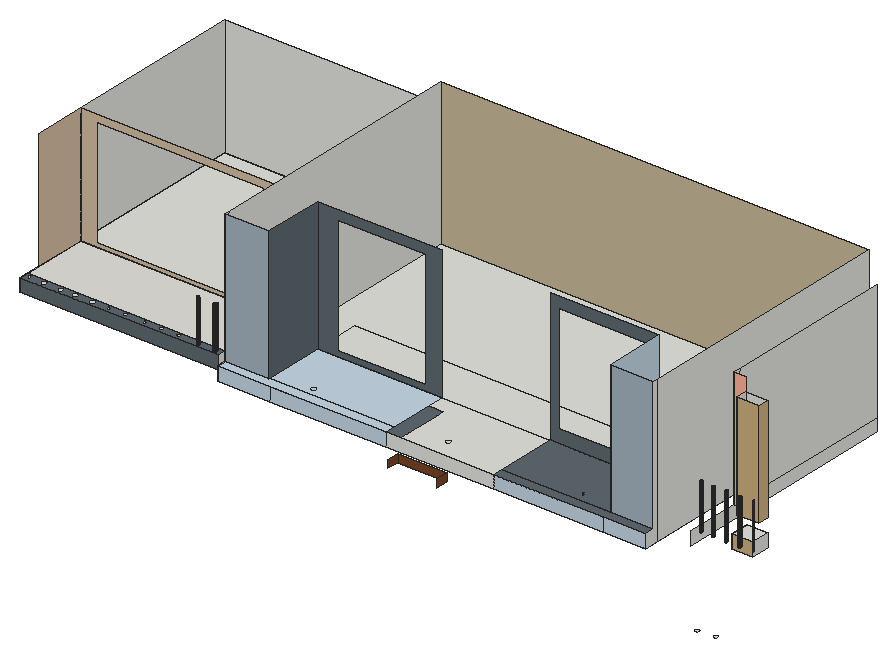
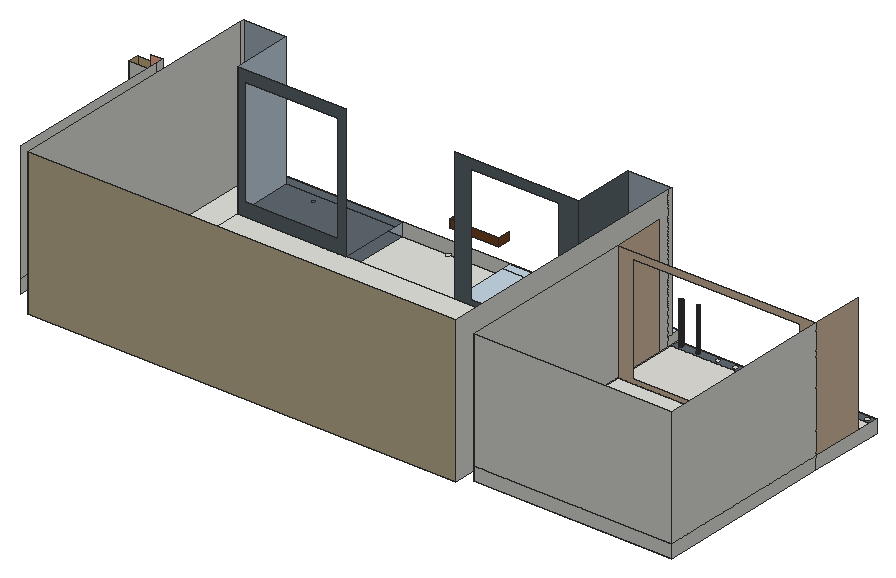
# SketchUp Ruby script. Lengths in inches.
U = 1.inch
M = Sketchup.active_model
def pt(a) = Geom::Point3d.new(a.map { |v| v * U })
def face(e, loops, mat)
  f = e.add_face(loops[0].map { |a| pt(a) })
  loops[1..].each { |l| e.add_face(l.map { |a| pt(a) }).erase! }
  f.material = f.back_material = mat if mat
  f
end
# faces: each face lists its corners as indices into pts; further lists are holes
def faces(e, pts, list, mat = nil) = list.each { |f| face(e, (f[0].is_a?(Array) ? f : [f]).map { |l| l.map { |i| pts[i] } }, mat) }
# xy, xz, yz: faces in a plane at the given z, y or x. An outline is a flat list of corners, or four numbers for a rectangle; further outlines are holes
def ring(l) = l.size == 4 ? [[l[0], l[1]], [l[2], l[1]], [l[2], l[3]], [l[0], l[3]]] : l.each_slice(2).to_a
def flat(e, list, mat, &to3) = list.each { |f| face(e, (f[0].is_a?(Array) ? f : [f]).map { |l| ring(l).map { |u, v| to3.(u, v) } }, mat) }
def xy(e, z, list, mat = nil) = flat(e, list, mat) { |x, y| [x, y, z] }
def xz(e, y, list, mat = nil) = flat(e, list, mat) { |x, z| [x, y, z] }
def yz(e, x, list, mat = nil) = flat(e, list, mat) { |y, z| [x, y, z] }
def lines(e, pts, list) = list.each { |a, b| e.add_line(pt(pts[a]), pt(pts[b])) }
# prism: a flat outline (further loops are holes) pulled along v
def prism(e, loops, v, mat = nil)
  f = face(e, loops, mat); d = Geom::Vector3d.new(v.map { |x| x * U })
  f.pushpull(f.normal.samedirection?(d) ? d.length : -d.length)
end
def box(e, o, s, mat = nil) = prism(e, [[o, [o[0] + s[0], o[1], o[2]], [o[0] + s[0], o[1] + s[1], o[2]], [o[0], o[1] + s[1], o[2]]]], [0, 0, s[2]], mat)
def at(x, y, z, deg = 0) = Geom::Transformation.translation(pt([x, y, z])) * Geom::Transformation.rotation(ORIGIN, Z_AXIS, deg.degrees)
def axes(o, x, y, z) = Geom::Transformation.new([*x, 0, *y, 0, *z, 0, *pt(o).to_a, 1])
def part(name) = M.definitions.add(name)
# library, detail: a bought-in or finely detailed component or shape, given as its bounding box
def library(name, o, s) = part(name).tap { |d| box(d.entities, o, s) }
def detail(e, o, s) = box(e.add_group.entities, o, s)
def put(e, d, t, mat = nil) = e.add_instance(d, t).tap { |i| i.material = mat if mat }
def group(e, t, mat = nil) = e.add_group.tap { |g| g.transformation = t; g.material = mat if mat }.entities
root = M.entities
M.materials.add("[Color B02]").color = [255, 178, 153]
M.materials.add("[Formica Laminate Dark]").color = [50, 53, 60]
M.materials.add("[Formica Laminate Light]").color = [213, 189, 164]
M.materials.add("[Formica Speckled Grey]").color = [94, 105, 111]
M.materials.add("[Marble Carrara Gold Floor Tile]").color = [225, 223, 217]
M.materials.add("[Quartz Light Brown]").color = [199, 184, 152]
M.materials.add("[Terrazzo Light Blue]1").color = [165, 180, 191]
M.materials.add("[Terrazzo Light Blue]2").color = [196, 214, 227]
M.materials.add("[Wood Floor Light]").color = [204, 176, 127]
M.materials.add("[Wood Veneer 01]2").color = [120, 70, 37]
xy(root,184.1875,[[619.39,128.83,619.78,128.89,620.14,129.04,620.45,129.27,620.6875,129.58,620.84,129.95,620.89,130.33,620.84,130.72,620.6875,131.08,620.45,131.4,620.14,131.63,619.78,131.78,619.39,131.83,619,131.78,618.64,131.63,618.33,131.4,618.09,131.08,617.9375,130.72,617.89,130.33,617.9375,129.95,618.09,129.58,618.33,129.27,618.64,129.04,619,128.89]])
xy(root,185.07,[[636.07,128.83,636.46,128.89,636.82,129.04,637.14,129.27,637.375,129.58,637.52,129.95,637.57,130.33,637.52,130.72,637.375,131.08,637.14,131.4,636.82,131.63,636.46,131.78,636.07,131.83,635.6875,131.78,635.32,131.63,635.01,131.4,634.78,131.08,634.625,130.72,634.57,130.33,634.625,129.95,634.78,129.58,635.01,129.27,635.32,129.04,635.6875,128.89]])
xy(root,236.59,[[622.89,165.2,641.83,182.57]])
xy(root,249,[[198.57,110.07,198.57,364.125,588.3,364.125,588.3,110.07,549.2,110.07,549.2,177.84,450.54,177.84,450.54,110.07,351.88,110.07,351.88,175.78,238.58,175.78,238.58,110.07],[9,122.79,189.57,191.15],[622.89,165.2,641.83,182.57],[9,191.15,189.57,355.125]])
xy(root,249,[[238.58,110.07,351.88,175.78],[450.54,110.07,549.2,177.84]],"[Formica Speckled Grey]")
xy(root,261,[[13.84,125.42,13.4,125.48,12.99,125.65,12.64,125.92,12.375,126.27,12.21,126.67,12.15,127.11,12.21,127.55,12.375,127.95,12.64,128.3,12.99,128.57,13.4,128.74,13.84,128.8,14.27,128.74,14.68,128.57,15.03,128.3,15.3,127.95,15.47,127.55,15.52,127.11,15.47,126.67,15.3,126.27,15.03,125.92,14.68,125.65,14.27,125.48],[27.09,125.42,26.65,125.48,26.24,125.65,25.89,125.92,25.625,126.27,25.46,126.67,25.4,127.11,25.46,127.55,25.625,127.95,25.89,128.3,26.24,128.57,26.65,128.74,27.09,128.8,27.52,128.74,27.93,128.57,28.28,128.3,28.55,127.95,28.72,127.55,28.77,127.11,28.72,126.67,28.55,126.27,28.28,125.92,27.93,125.65,27.52,125.48],[42.4,125.42,41.96,125.48,41.56,125.65,41.21,125.92,40.9375,126.27,40.77,126.67,40.71,127.11,40.77,127.55,40.9375,127.95,41.21,128.3,41.56,128.57,41.96,128.74,42.4,128.8,42.84,128.74,43.24,128.57,43.59,128.3,43.86,127.95,44.03,127.55,44.09,127.11,44.03,126.67,43.86,126.27,43.59,125.92,43.24,125.65,42.84,125.48],[55.4,125.42,54.96,125.48,54.56,125.65,54.21,125.92,53.9375,126.27,53.77,126.67,53.71,127.11,53.77,127.55,53.9375,127.95,54.21,128.3,54.56,128.57,54.96,128.74,55.4,128.8,55.84,128.74,56.24,128.57,56.59,128.3,56.86,127.95,57.03,127.55,57.09,127.11,57.03,126.67,56.86,126.27,56.59,125.92,56.24,125.65,55.84,125.48],[71.27,125.42,70.84,125.48,70.43,125.65,70.08,125.92,69.8125,126.27,69.64,126.67,69.59,127.11,69.64,127.55,69.8125,127.95,70.08,128.3,70.43,128.57,70.84,128.74,71.27,128.8,71.71,128.74,72.12,128.57,72.47,128.3,72.74,127.95,72.9,127.55,72.96,127.11,72.9,126.67,72.74,126.27,72.47,125.92,72.12,125.65,71.71,125.48],
  [86.21,125.42,85.78,125.48,85.37,125.65,85.02,125.92,84.75,126.27,84.58,126.67,84.52,127.11,84.58,127.55,84.75,127.95,85.02,128.3,85.37,128.57,85.78,128.74,86.21,128.8,86.65,128.74,87.06,128.57,87.41,128.3,87.67,127.95,87.84,127.55,87.9,127.11,87.84,126.67,87.67,126.27,87.41,125.92,87.06,125.65,86.65,125.48],[101.27,125.42,100.84,125.48,100.43,125.65,100.08,125.92,99.8125,126.27,99.64,126.67,99.59,127.11,99.64,127.55,99.8125,127.95,100.08,128.3,100.43,128.57,100.84,128.74,101.27,128.8,101.71,128.74,102.12,128.57,102.47,128.3,102.74,127.95,102.9,127.55,102.96,127.11,102.9,126.67,102.74,126.27,102.47,125.92,102.12,125.65,101.71,125.48],[118.77,125.42,118.34,125.48,117.93,125.65,117.58,125.92,117.3125,126.27,117.14,126.67,117.09,127.11,117.14,127.55,117.3125,127.95,117.58,128.3,117.93,128.57,118.34,128.74,118.77,128.8,119.21,128.74,119.62,128.57,119.97,128.3,120.24,127.95,120.4,127.55,120.46,127.11,120.4,126.67,120.24,126.27,119.97,125.92,119.62,125.65,119.21,125.48],[133.84,125.42,133.4,125.48,132.99,125.65,132.64,125.92,132.375,126.27,132.21,126.67,132.15,127.11,132.21,127.55,132.375,127.95,132.64,128.3,132.99,128.57,133.4,128.74,133.84,128.8,134.27,128.74,134.68,128.57,135.03,128.3,135.3,127.95,135.47,127.55,135.52,127.11,135.47,126.67,135.3,126.27,135.03,125.92,134.68,125.65,134.27,125.48],[149.84,125.42,149.4,125.48,148.99,125.65,148.64,125.92,148.375,126.27,148.21,126.67,148.15,127.11,148.21,127.55,148.375,127.95,148.64,128.3,148.99,128.57,149.4,128.74,149.84,128.8,150.27,128.74,150.68,128.57,151.03,128.3,151.3,127.95,151.47,127.55,151.52,127.11,151.47,126.67,151.3,126.27,151.03,125.92,150.68,125.65,150.27,125.48],
  [167.96,125.42,167.53,125.48,167.12,125.65,166.77,125.92,166.5,126.27,166.33,126.67,166.27,127.11,166.33,127.55,166.5,127.95,166.77,128.3,167.12,128.57,167.53,128.74,167.96,128.8,168.4,128.74,168.81,128.57,169.16,128.3,169.42,127.95,169.59,127.55,169.65,127.11,169.59,126.67,169.42,126.27,169.16,125.92,168.81,125.65,168.4,125.48],[183.34,125.42,182.9,125.48,182.49,125.65,182.14,125.92,181.875,126.27,181.71,126.67,181.65,127.11,181.71,127.55,181.875,127.95,182.14,128.3,182.49,128.57,182.9,128.74,183.34,128.8,183.77,128.74,184.18,128.57,184.53,128.3,184.8,127.95,184.97,127.55,185.02,127.11,184.97,126.67,184.8,126.27,184.53,125.92,184.18,125.65,183.77,125.48],[395.34,125.42,395.77,125.48,396.18,125.65,396.53,125.92,396.8,126.27,396.97,126.67,397.02,127.11,396.97,127.55,396.8,127.95,396.53,128.3,396.18,128.57,395.77,128.74,395.34,128.8,394.9,128.74,394.49,128.57,394.14,128.3,393.875,127.95,393.71,127.55,393.65,127.11,393.71,126.67,393.875,126.27,394.14,125.92,394.49,125.65,394.9,125.48],[617.36,136.16,617.06,136.2,616.77,136.32,616.52,136.51,616.34,136.76,616.22,137.04,616.18,137.35,616.22,137.66,616.34,137.94,616.52,138.19,616.77,138.38,617.06,138.5,617.36,138.54,617.67,138.5,617.96,138.38,618.2,138.19,618.39,137.94,618.51,137.66,618.55,137.35,618.51,137.04,618.39,136.76,618.2,136.51,617.96,136.32,617.67,136.2],[628.3,136.16,627.99,136.2,627.71,136.32,627.46,136.51,627.27,136.76,627.16,137.04,627.11,137.35,627.16,137.66,627.27,137.94,627.46,138.19,627.71,138.38,627.99,138.5,628.3,138.54,628.61,138.5,628.9,138.38,629.14,138.19,629.33,137.94,629.45,137.66,629.49,137.35,629.45,137.04,629.33,136.76,629.14,136.51,628.9,136.32,628.61,136.2],
  [640.36,136.16,640.06,136.2,639.77,136.32,639.52,136.51,639.34,136.76,639.22,137.04,639.18,137.35,639.22,137.66,639.34,137.94,639.52,138.19,639.77,138.38,640.06,138.5,640.36,138.54,640.67,138.5,640.96,138.38,641.2,138.19,641.39,137.94,641.51,137.66,641.55,137.35,641.51,137.04,641.39,136.76,641.2,136.51,640.96,136.32,640.67,136.2],[652.55,136.16,652.24,136.2,651.96,136.32,651.71,136.51,651.52,136.76,651.41,137.04,651.36,137.35,651.41,137.66,651.52,137.94,651.71,138.19,651.96,138.38,652.24,138.5,652.55,138.54,652.86,138.5,653.15,138.38,653.39,138.19,653.58,137.94,653.7,137.66,653.74,137.35,653.7,137.04,653.58,136.76,653.39,136.51,653.15,136.32,652.86,136.2],[621.3,172.64,641.63,182.57],[238.58,174.4375,549.2,216.55],[9,191.15,189.57,355.125]])
xy(root,261,[[450.54,110.07,588.3,119.07],[[450.54,119.07,549.2,174.4375],[518.09,125.42,517.65,125.48,517.24,125.65,516.89,125.92,516.625,126.27,516.46,126.67,516.4,127.11,516.46,127.55,516.625,127.95,516.89,128.3,517.24,128.57,517.65,128.74,518.09,128.8,518.52,128.74,518.93,128.57,519.28,128.3,519.55,127.95,519.72,127.55,519.77,127.11,519.72,126.67,519.55,126.27,519.28,125.92,518.93,125.65,518.52,125.48]],[[9,122.79,189.57,130.88],[183.34,125.42,182.9,125.48,182.49,125.65,182.14,125.92,181.875,126.27,181.71,126.67,181.65,127.11,181.71,127.55,181.875,127.95,182.14,128.3,182.49,128.57,182.9,128.74,183.34,128.8,183.77,128.74,184.18,128.57,184.53,128.3,184.8,127.95,184.97,127.55,185.02,127.11,184.97,126.67,184.8,126.27,184.53,125.92,184.18,125.65,183.77,125.48],[13.84,125.42,13.4,125.48,12.99,125.65,12.64,125.92,12.375,126.27,12.21,126.67,12.15,127.11,12.21,127.55,12.375,127.95,12.64,128.3,12.99,128.57,13.4,128.74,13.84,128.8,14.27,128.74,14.68,128.57,15.03,128.3,15.3,127.95,15.47,127.55,15.52,127.11,15.47,126.67,15.3,126.27,15.03,125.92,14.68,125.65,14.27,125.48],[167.96,125.42,167.53,125.48,167.12,125.65,166.77,125.92,166.5,126.27,166.33,126.67,166.27,127.11,166.33,127.55,166.5,127.95,166.77,128.3,167.12,128.57,167.53,128.74,167.96,128.8,168.4,128.74,168.81,128.57,169.16,128.3,169.42,127.95,169.59,127.55,169.65,127.11,169.59,126.67,169.42,126.27,169.16,125.92,168.81,125.65,168.4,125.48],[27.09,125.42,26.65,125.48,26.24,125.65,25.89,125.92,25.625,126.27,25.46,126.67,25.4,127.11,25.46,127.55,25.625,127.95,25.89,128.3,26.24,128.57,26.65,128.74,27.09,128.8,27.52,128.74,27.93,128.57,28.28,128.3,28.55,127.95,28.72,127.55,28.77,127.11,28.72,126.67,28.55,126.27,28.28,125.92,27.93,125.65,27.52,125.48],[149.84,125.42,149.4,125.48,148.99,125.65,148.64,125.92,148.375,126.27,148.21,126.67,148.15,127.11,148.21,127.55,148.375,127.95,148.64,128.3,148.99,128.57,149.4,128.74,149.84,128.8,150.27,128.74,150.68,128.57,151.03,128.3,151.3,127.95,151.47,127.55,151.52,127.11,151.47,126.67,151.3,126.27,151.03,125.92,150.68,125.65,150.27,125.48],[42.4,125.42,41.96,125.48,41.56,125.65,41.21,125.92,40.9375,126.27,40.77,126.67,40.71,127.11,40.77,127.55,40.9375,127.95,41.21,128.3,41.56,128.57,41.96,128.74,42.4,128.8,42.84,128.74,43.24,128.57,43.59,128.3,43.86,127.95,44.03,127.55,44.09,127.11,44.03,126.67,43.86,126.27,43.59,125.92,43.24,125.65,42.84,125.48],[133.84,125.42,133.4,125.48,132.99,125.65,132.64,125.92,132.375,126.27,132.21,126.67,132.15,127.11,132.21,127.55,132.375,127.95,132.64,128.3,132.99,128.57,133.4,128.74,133.84,128.8,134.27,128.74,134.68,128.57,135.03,128.3,135.3,127.95,135.47,127.55,135.52,127.11,135.47,126.67,135.3,126.27,135.03,125.92,134.68,125.65,134.27,125.48],[55.4,125.42,54.96,125.48,54.56,125.65,54.21,125.92,53.9375,126.27,53.77,126.67,53.71,127.11,53.77,127.55,53.9375,127.95,54.21,128.3,54.56,128.57,54.96,128.74,55.4,128.8,55.84,128.74,56.24,128.57,56.59,128.3,56.86,127.95,57.03,127.55,57.09,127.11,57.03,126.67,56.86,126.27,56.59,125.92,56.24,125.65,55.84,125.48],[118.77,125.42,118.34,125.48,117.93,125.65,117.58,125.92,117.3125,126.27,117.14,126.67,117.09,127.11,117.14,127.55,117.3125,127.95,117.58,128.3,117.93,128.57,118.34,128.74,118.77,128.8,119.21,128.74,119.62,128.57,119.97,128.3,120.24,127.95,120.4,127.55,120.46,127.11,120.4,126.67,120.24,126.27,119.97,125.92,119.62,125.65,119.21,125.48],[71.27,125.42,70.84,125.48,70.43,125.65,70.08,125.92,69.8125,126.27,69.64,126.67,69.59,127.11,69.64,127.55,69.8125,127.95,70.08,128.3,70.43,128.57,70.84,128.74,71.27,128.8,71.71,128.74,72.12,128.57,72.47,128.3,72.74,127.95,72.9,127.55,72.96,127.11,72.9,126.67,72.74,126.27,72.47,125.92,72.12,125.65,71.71,125.48],[101.27,125.42,100.84,125.48,100.43,125.65,100.08,125.92,99.8125,126.27,99.64,126.67,99.59,127.11,99.64,127.55,99.8125,127.95,100.08,128.3,100.43,128.57,100.84,128.74,101.27,128.8,101.71,128.74,102.12,128.57,102.47,128.3,102.74,127.95,102.9,127.55,102.96,127.11,102.9,126.67,102.74,126.27,102.47,125.92,102.12,125.65,101.71,125.48],[86.21,125.42,85.78,125.48,85.37,125.65,85.02,125.92,84.75,126.27,84.58,126.67,84.52,127.11,84.58,127.55,84.75,127.95,85.02,128.3,85.37,128.57,85.78,128.74,86.21,128.8,86.65,128.74,87.06,128.57,87.41,128.3,87.67,127.95,87.84,127.55,87.9,127.11,87.84,126.67,87.67,126.27,87.41,125.92,87.06,125.65,86.65,125.48]],[518.09,125.42,518.52,125.48,518.93,125.65,519.28,125.92,519.55,126.27,519.72,126.67,519.77,127.11,519.72,127.55,519.55,127.95,519.28,128.3,518.93,128.57,518.52,128.74,518.09,128.8,517.65,128.74,517.24,128.57,516.89,128.3,516.625,127.95,516.46,127.55,516.4,127.11,516.46,126.67,516.625,126.27,516.89,125.92,517.24,125.65,517.65,125.48]],"[Formica Speckled Grey]")
xy(root,261,[[9,130.88,189.57,191.15]],"[Marble Carrara Gold Floor Tile]")
xy(root,261,[[198.57,110.07,351.88,119.07],[[238.58,119.07,351.88,174.4375],[272.59,125.42,272.15,125.48,271.74,125.65,271.39,125.92,271.125,126.27,270.96,126.67,270.9,127.11,270.96,127.55,271.125,127.95,271.39,128.3,271.74,128.57,272.15,128.74,272.59,128.8,273.02,128.74,273.43,128.57,273.78,128.3,274.05,127.95,274.22,127.55,274.27,127.11,274.22,126.67,274.05,126.27,273.78,125.92,273.43,125.65,273.02,125.48]],[272.59,125.42,273.02,125.48,273.43,125.65,273.78,125.92,274.05,126.27,274.22,126.67,274.27,127.11,274.22,127.55,274.05,127.95,273.78,128.3,273.43,128.57,273.02,128.74,272.59,128.8,272.15,128.74,271.74,128.57,271.39,128.3,271.125,127.95,270.96,127.55,270.9,127.11,270.96,126.67,271.125,126.27,271.39,125.92,271.74,125.65,272.15,125.48]],"[Terrazzo Light Blue]2")
xz(root,88.2,[[380.3,255.83,424.94,262.65]],"[Wood Veneer 01]2")
xz(root,110.07,[[351.88,249,450.54,261]])
xz(root,110.07,[[198.57,249,246.77,261],[246.77,249,351.88,261],[450.54,249,549.2,261],[549.2,249,588.3,261]],"[Terrazzo Light Blue]2")
xz(root,119.07,[[198.57,261,238.58,381],[549.2,261,588.3,381]],"[Terrazzo Light Blue]1")
xz(root,122.79,[[9,249,189.57,261]],"[Formica Speckled Grey]")
xz(root,165.2,[[622.89,236.59,641.83,249]],"[Wood Floor Light]")
xz(root,172.64,[[621.3,261,641.63,356.625]],"[Wood Floor Light]")
xz(root,174.4375,[[[238.58,261,351.88,381],[256.64,265.55,336.77,372.68]],[[450.54,261,549.2,381],[458.21,273.03,542.42,371.125]]],"[Formica Speckled Grey]")
xz(root,182.57,[[622.89,236.59,641.83,249],[621.3,261,641.63,356.625]])
xz(root,182.57,[[611.125,261,621.3,369]],"[Color B02]")
xz(root,191.15,[[9,249,189.57,261]])
xz(root,191.15,[[[9,261,189.57,369],[24.08,264.5,176.08,363]]],"[Formica Laminate Light]")
xz(root,355.125,[[9,249,189.57,261],[9,261,189.57,369]])
xz(root,364.125,[[198.57,249,588.3,381]],"[Quartz Light Brown]")
yz(root,9,[[122.79,249,191.15,261],[191.15,249,355.125,261],[191.15,261,355.125,369]])
yz(root,9,[[144.21,261,191.15,369]],"[Formica Laminate Light]")
yz(root,189.57,[[122.79,249,191.15,261],[191.15,249,355.125,261],[191.15,261,355.125,369]])
yz(root,189.57,[[144.21,261,191.15,369]],"[Formica Laminate Light]")
yz(root,198.57,[[110.07,249,122.79,261],[122.79,249,364.125,381],[119.07,261,122.79,381]])
yz(root,238.58,[[119.07,261,174.4375,381]],"[Formica Speckled Grey]")
yz(root,380.3,[[77.26,255.83,88.2,262.65]],"[Wood Veneer 01]2")
yz(root,424.94,[[77.26,255.83,88.2,262.65]],"[Wood Veneer 01]2")
yz(root,549.2,[[119.07,261,174.4375,381]],"[Terrazzo Light Blue]2")
yz(root,588.3,[[110.07,249,122.79,249,122.79,381,119.07,381,119.07,261,110.07,261],[122.79,249,364.125,381]])
yz(root,611.125,[[133.3,249,344.36,249,344.36,261,189.24,261,189.24,369,182.57,369,182.57,261,133.3,261],[189.24,261,344.36,369]])
yz(root,621.3,[[172.64,261,182.57,356.625]])
yz(root,622.89,[[165.2,236.59,182.57,249]],"[Wood Floor Light]")
yz(root,641.63,[[172.64,261,182.57,356.625]],"[Wood Floor Light]")
yz(root,641.83,[[165.2,236.59,182.57,249]])
p = [[167.53,125.48,261],[167.96,125.42,261],[167.96,125.42,298.84],[167.53,125.48,298.84],[168.4,125.48,261],[168.4,125.48,298.84],
  [182.9,125.48,261],[183.34,125.42,261],[183.34,125.42,298.84],[182.9,125.48,298.84],[183.77,125.48,261],[183.77,125.48,298.84],
  [167.12,125.65,261],[167.12,125.65,298.84],[168.81,125.65,261],[168.81,125.65,298.84],[182.49,125.65,261],[182.49,125.65,298.84],
  [184.18,125.65,261],[184.18,125.65,298.84],[166.77,125.92,261],[166.77,125.92,298.84],[169.16,125.92,261],[169.16,125.92,298.84],
  [182.14,125.92,261],[182.14,125.92,298.84],[184.53,125.92,261],[184.53,125.92,298.84],[166.5,126.27,261],[166.5,126.27,298.84],
  [169.42,126.27,261],[169.42,126.27,298.84],[181.875,126.27,261],[181.875,126.27,298.84],[184.8,126.27,261],[184.8,126.27,298.84],
  [166.33,126.67,261],[166.33,126.67,298.84],[169.59,126.67,261],[169.59,126.67,298.84],[181.71,126.67,261],[181.71,126.67,298.84],
  [184.97,126.67,261],[184.97,126.67,298.84],[166.27,127.11,261],[166.27,127.11,298.84],[181.65,127.11,261],[181.65,127.11,298.84],
  [185.02,127.11,261],[185.02,127.11,298.84],[166.33,127.55,261],[166.33,127.55,298.84],[181.71,127.55,261],[181.71,127.55,298.84],
  [184.97,127.55,261],[184.97,127.55,298.84],[166.5,127.95,261],[166.5,127.95,298.84],[181.875,127.95,261],[181.875,127.95,298.84],
  [184.8,127.95,261],[184.8,127.95,298.84],[166.77,128.3,261],[166.77,128.3,298.84],[182.14,128.3,261],[182.14,128.3,298.84],
  [184.53,128.3,261],[184.53,128.3,298.84],[167.12,128.57,261],[167.12,128.57,298.84],[182.49,128.57,261],[182.49,128.57,298.84],
  [184.18,128.57,261],[184.18,128.57,298.84],[182.9,128.74,261],[182.9,128.74,298.84],[183.77,128.74,261],[183.77,128.74,298.84],
  [183.34,128.8,261],[183.34,128.8,298.84],[616.77,136.32,261],[617.06,136.2,261],[617.06,136.2,302.22],[616.77,136.32,302.22],
  [617.36,136.16,261],[617.36,136.16,302.22],[617.67,136.2,261],[617.67,136.2,302.22],[617.96,136.32,261],[617.96,136.32,302.22],
  [627.71,136.32,261],[627.99,136.2,261],[627.99,136.2,301.8125],[627.71,136.32,301.8125],[628.3,136.16,261],[628.3,136.16,301.8125],
  [628.61,136.2,261],[628.61,136.2,301.8125],[628.9,136.32,261],[628.9,136.32,301.8125],[639.77,136.32,261],[640.06,136.2,261],
  [640.06,136.2,302.3125],[639.77,136.32,302.3125],[640.36,136.16,261],[640.36,136.16,302.3125],[640.67,136.2,261],[640.67,136.2,302.3125],
  [640.96,136.32,261],[640.96,136.32,302.3125],[651.96,136.32,261],[652.24,136.2,261],[652.24,136.2,301.91],[651.96,136.32,301.91],
  [652.55,136.16,261],[652.55,136.16,301.91],[652.86,136.2,261],[652.86,136.2,301.91],[653.15,136.32,261],[653.15,136.32,301.91],
  [616.52,136.51,261],[616.52,136.51,302.22],[618.2,136.51,261],[618.2,136.51,302.22],[627.46,136.51,261],[627.46,136.51,301.8125],
  [629.14,136.51,261],[629.14,136.51,301.8125],[639.52,136.51,261],[639.52,136.51,302.3125],[641.2,136.51,261],[641.2,136.51,302.3125],
  [651.71,136.51,261],[651.71,136.51,301.91],[653.39,136.51,261],[653.39,136.51,301.91],[616.34,136.76,261],[616.34,136.76,302.22],
  [618.39,136.76,261],[618.39,136.76,302.22],[627.27,136.76,261],[627.27,136.76,301.8125],[629.33,136.76,261],[629.33,136.76,301.8125],
  [639.34,136.76,261],[639.34,136.76,302.3125],[641.39,136.76,261],[641.39,136.76,302.3125],[651.52,136.76,261],[651.52,136.76,301.91],
  [653.58,136.76,261],[653.58,136.76,301.91],[616.22,137.04,261],[616.26,136.9375,302.22],[616.22,137.04,302.22],[618.51,137.04,261],
  [618.51,137.04,302.22],[618.47,136.9375,302.22],[627.16,137.04,261],[627.16,137.04,301.8125],[629.45,137.04,261],[629.45,137.04,301.8125],
  [639.22,137.04,261],[639.22,137.04,302.3125],[641.51,137.04,261],[641.51,137.04,302.3125],[651.41,137.04,261],[651.47,136.9,301.91],
  [651.41,137.04,301.91],[653.7,137.04,261],[653.7,137.04,301.91],[653.64,136.9,301.91],[664.22,137.04,261],[664.34,136.76,261],
  [664.34,136.76,302.8125],[664.22,137.04,302.8125],[616.18,137.35,261],[616.18,137.35,302.22],[618.55,137.35,261],[618.55,137.35,302.22],
  [627.11,137.35,261],[627.11,137.35,301.8125],[629.49,137.35,261],[629.49,137.35,301.8125],[639.18,137.35,261],[639.18,137.35,302.3125],
  [641.55,137.35,261],[641.55,137.35,302.3125],[651.36,137.35,261],[651.36,137.35,301.91],[653.74,137.35,261],[653.74,137.35,301.91],
  [664.18,137.35,261],[664.18,137.35,302.8125],[616.22,137.66,261],[616.22,137.66,302.22],[618.51,137.66,261],[618.51,137.66,302.22],
  [627.16,137.66,261],[627.16,137.66,301.8125],[629.45,137.66,261],[629.45,137.66,301.8125],[639.22,137.66,261],[639.22,137.66,302.3125],
  [641.51,137.66,261],[641.51,137.66,302.3125],[651.41,137.66,261],[651.41,137.66,301.91],[653.7,137.66,261],[653.7,137.66,301.91],
  [664.22,137.66,261],[664.22,137.66,302.8125],[616.34,137.94,261],[616.34,137.94,302.22],[618.39,137.94,261],[618.39,137.94,302.22],
  [627.27,137.94,261],[627.27,137.94,301.8125],[629.33,137.94,261],[629.33,137.94,301.8125],[639.34,137.94,261],[639.34,137.94,302.3125],
  [641.39,137.94,261],[641.39,137.94,302.3125],[651.52,137.94,261],[651.52,137.94,301.91],[653.58,137.94,261],[653.58,137.94,301.91],
  [664.34,137.94,261],[664.34,137.94,302.8125],[616.52,138.19,261],[616.52,138.19,302.22],[618.2,138.19,261],[618.2,138.19,302.22],
  [627.46,138.19,261],[627.46,138.19,301.8125],[629.14,138.19,261],[629.14,138.19,301.8125],[639.52,138.19,261],[639.52,138.19,302.3125],
  [641.2,138.19,261],[641.2,138.19,302.3125],[651.71,138.19,261],[651.71,138.19,301.91],[653.39,138.19,261],[653.39,138.19,301.91],
  [616.77,138.38,261],[616.77,138.38,302.22],[617.96,138.38,261],[617.96,138.38,302.22],[627.71,138.38,261],[627.71,138.38,301.8125],
  [628.9,138.38,261],[628.9,138.38,301.8125],[639.77,138.38,261],[639.77,138.38,302.3125],[640.96,138.38,261],[640.96,138.38,302.3125],
  [651.96,138.38,261],[651.96,138.38,301.91],[653.15,138.38,261],[653.15,138.38,301.91],[617.06,138.5,261],[617.06,138.5,302.22],
  [617.67,138.5,261],[617.67,138.5,302.22],[627.99,138.5,261],[627.99,138.5,301.8125],[628.61,138.5,261],[628.61,138.5,301.8125],
  [640.06,138.5,261],[640.06,138.5,302.3125],[640.67,138.5,261],[640.67,138.5,302.3125],[652.24,138.5,261],[652.24,138.5,301.91],
  [652.86,138.5,261],[652.86,138.5,301.91],[617.36,138.54,261],[617.36,138.54,302.22],[628.3,138.54,261],[628.3,138.54,301.8125],
  [640.36,138.54,261],[640.36,138.54,302.3125],[652.55,138.54,261],[652.55,138.54,301.91]]
faces(root,p,[[0,1,2,3],[1,4,5,2],[6,7,8,9],[7,10,11,8],[12,0,3,13],[4,14,15,5],[16,6,9,17],[10,18,19,11],
  [20,12,13,21],[14,22,23,15],[24,16,17,25],[18,26,27,19],[28,20,21,29],[22,30,31,23],[32,24,25,33],[26,34,35,27],
  [36,28,29,37],[30,38,39,31],[40,32,33,41],[34,42,43,35],[44,36,37,45],[46,40,41,47],[42,48,49,43],[50,44,45,51],
  [52,46,47,53],[48,54,55,49],[56,50,51,57],[58,52,53,59],[54,60,61,55],[62,56,57,63],[64,58,59,65],[60,66,67,61],
  [68,62,63,69],[70,64,65,71],[66,72,73,67],[74,70,71,75],[72,76,77,73],[78,74,75,79],[76,78,79,77],[80,81,82,83],
  [81,84,85,82],[84,86,87,85],[86,88,89,87],[90,91,92,93],[91,94,95,92],[94,96,97,95],[96,98,99,97],[100,101,102,103],
  [101,104,105,102],[104,106,107,105],[106,108,109,107],[110,111,112,113],[111,114,115,112],[114,116,117,115],[116,118,119,117],[120,80,83,121],
  [88,122,123,89],[124,90,93,125],[98,126,127,99],[128,100,103,129],[108,130,131,109],[132,110,113,133],[118,134,135,119],[136,120,121,137],
  [122,138,139,123],[140,124,125,141],[126,142,143,127],[144,128,129,145],[130,146,147,131],[148,132,133,149],[134,150,151,135],[152,136,137,153,154],
  [138,155,156,157,139],[158,140,141,159],[142,160,161,143],[162,144,145,163],[146,164,165,147],[166,148,149,167,168],[150,169,170,171,151],[172,173,174,175],
  [176,152,154,177],[155,178,179,156],[180,158,159,181],[160,182,183,161],[184,162,163,185],[164,186,187,165],[188,166,168,189],[169,190,191,170],
  [192,172,175,193],[194,176,177,195],[178,196,197,179],[198,180,181,199],[182,200,201,183],[202,184,185,203],[186,204,205,187],[206,188,189,207],
  [190,208,209,191],[210,192,193,211],[212,194,195,213],[196,214,215,197],[216,198,199,217],[200,218,219,201],[220,202,203,221],[204,222,223,205],
  [224,206,207,225],[208,226,227,209],[228,210,211,229],[230,212,213,231],[214,232,233,215],[234,216,217,235],[218,236,237,219],[238,220,221,239],
  [222,240,241,223],[242,224,225,243],[226,244,245,227],[246,230,231,247],[232,248,249,233],[250,234,235,251],[236,252,253,237],[254,238,239,255],
  [240,256,257,241],[258,242,243,259],[244,260,261,245],[262,246,247,263],[248,264,265,249],[266,250,251,267],[252,268,269,253],[270,254,255,271],
  [256,272,273,257],[274,258,259,275],[260,276,277,261],[278,262,263,279],[264,278,279,265],[280,266,267,281],[268,280,281,269],[282,270,271,283],
  [272,282,283,273],[284,274,275,285],[276,284,285,277]],"[Formica Laminate Dark]")
